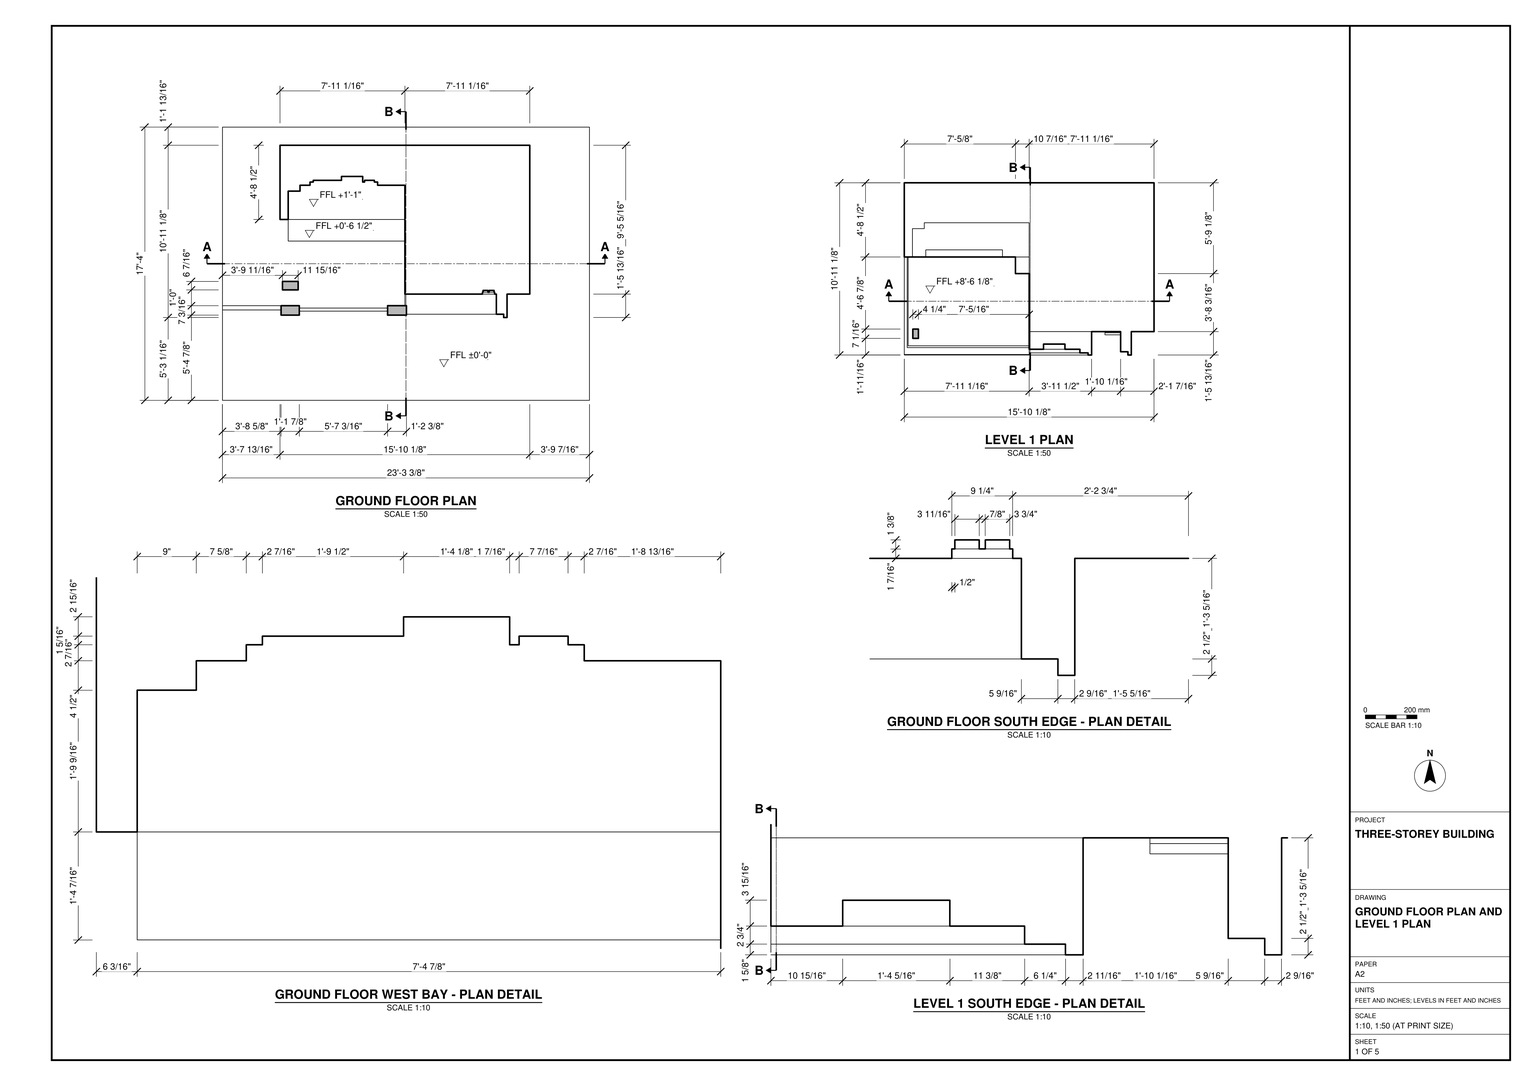
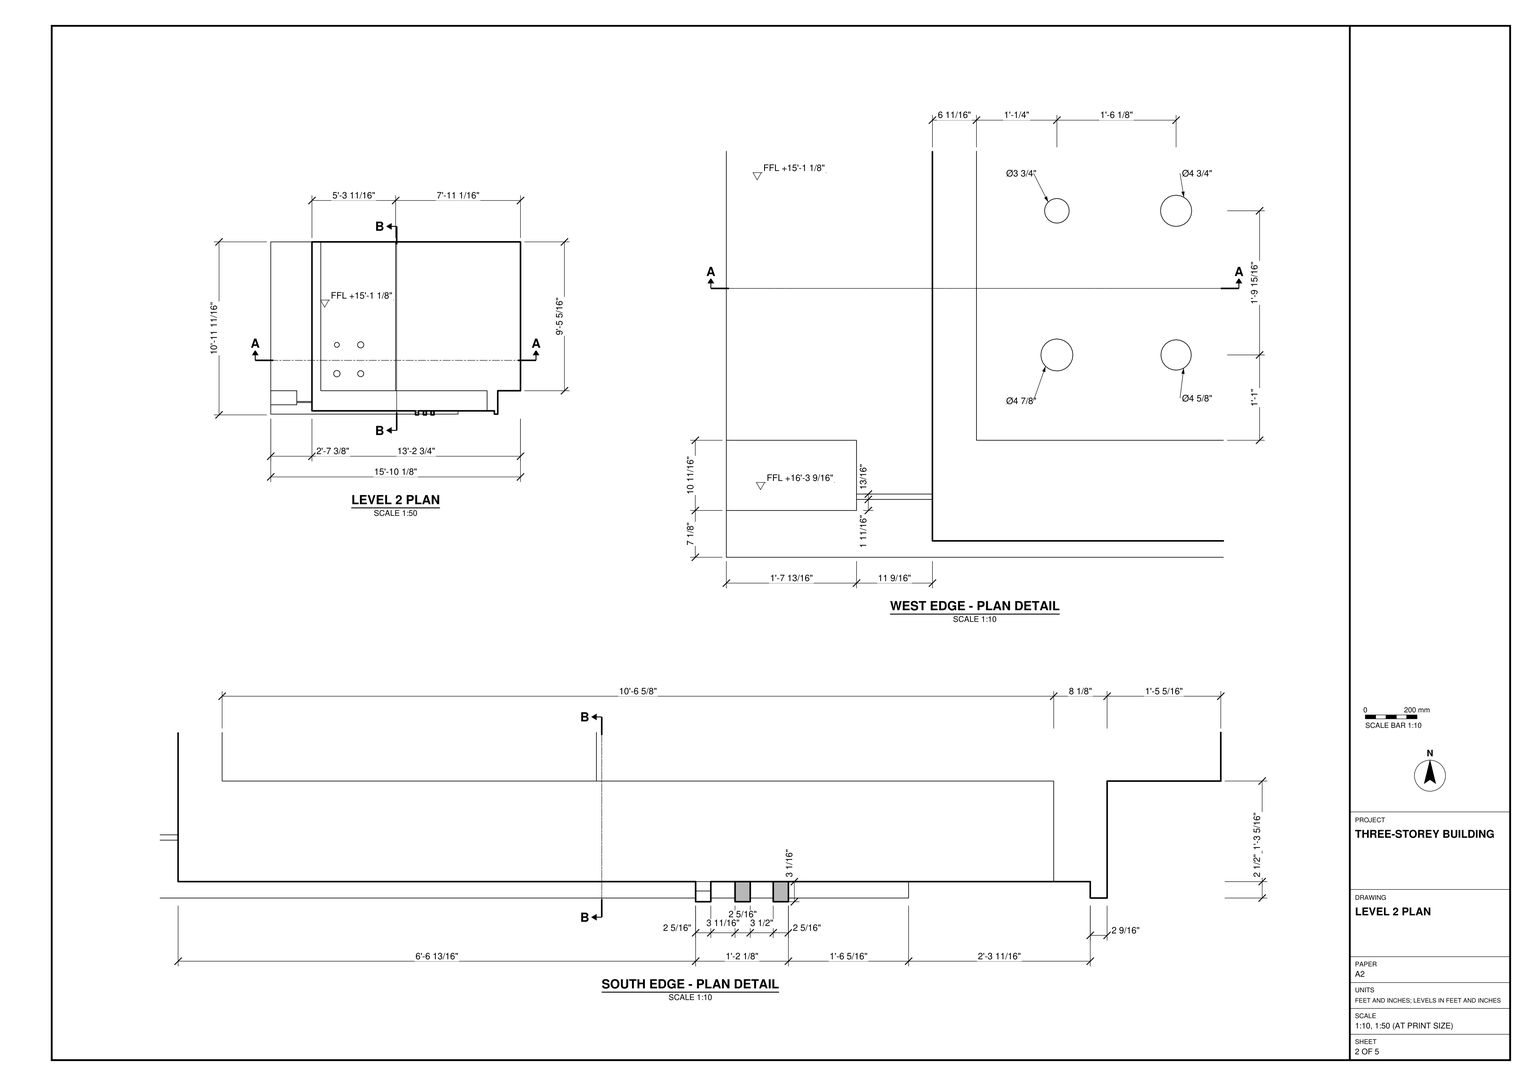
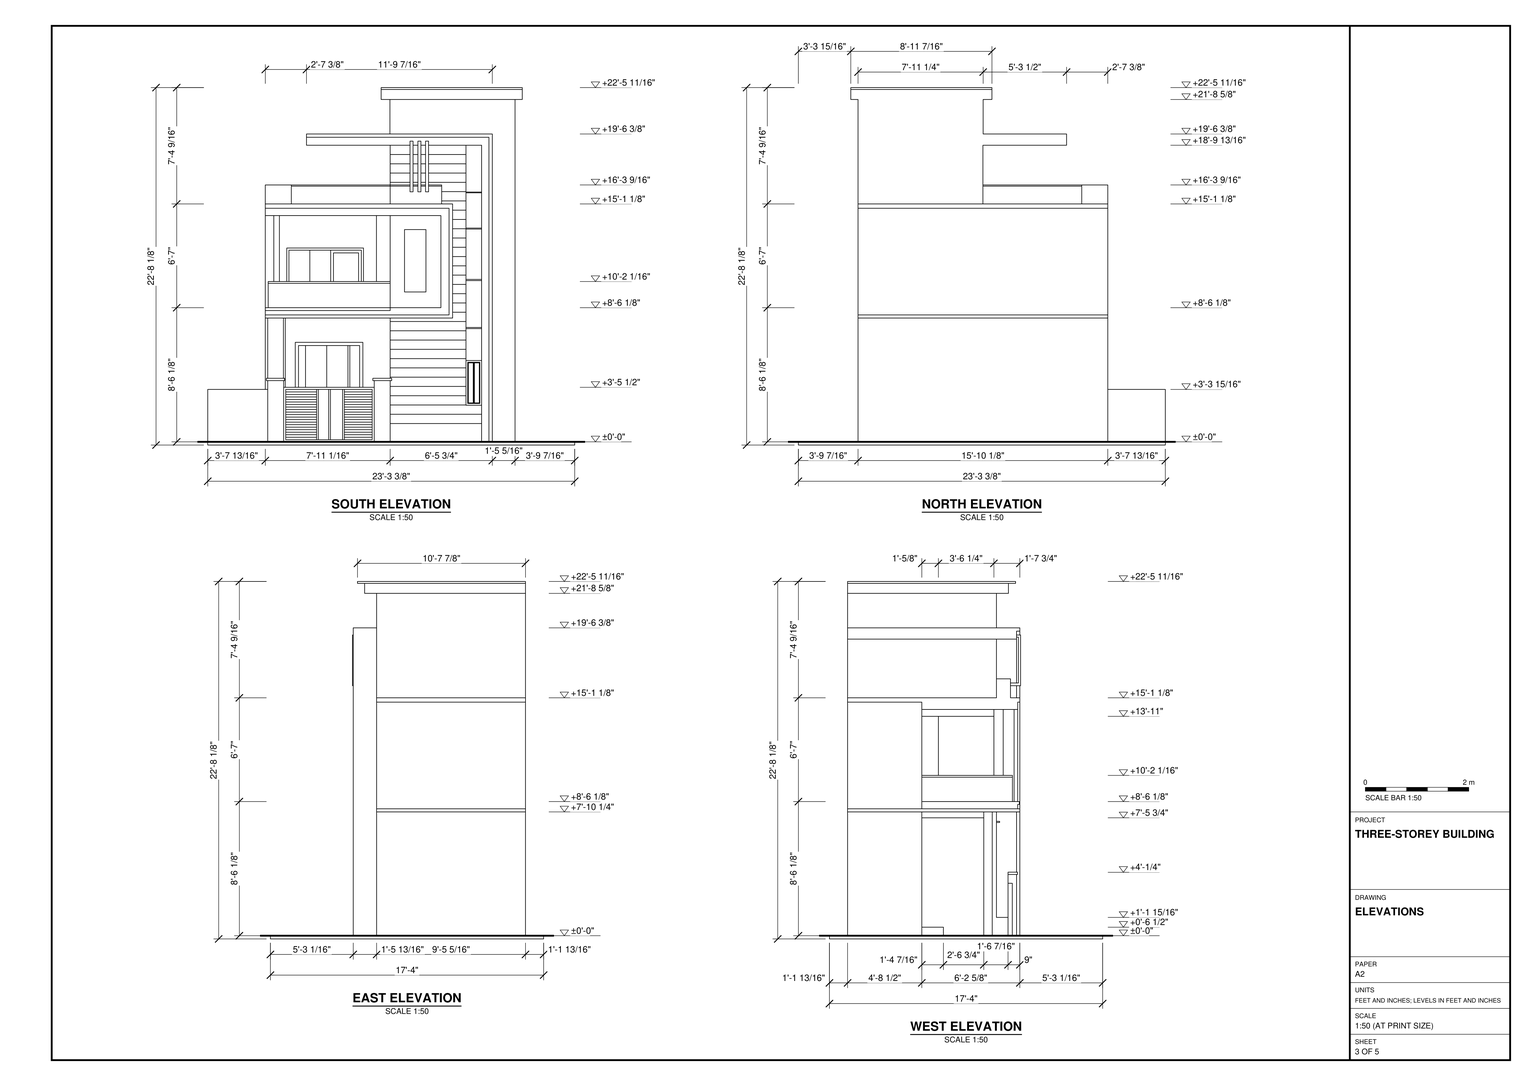
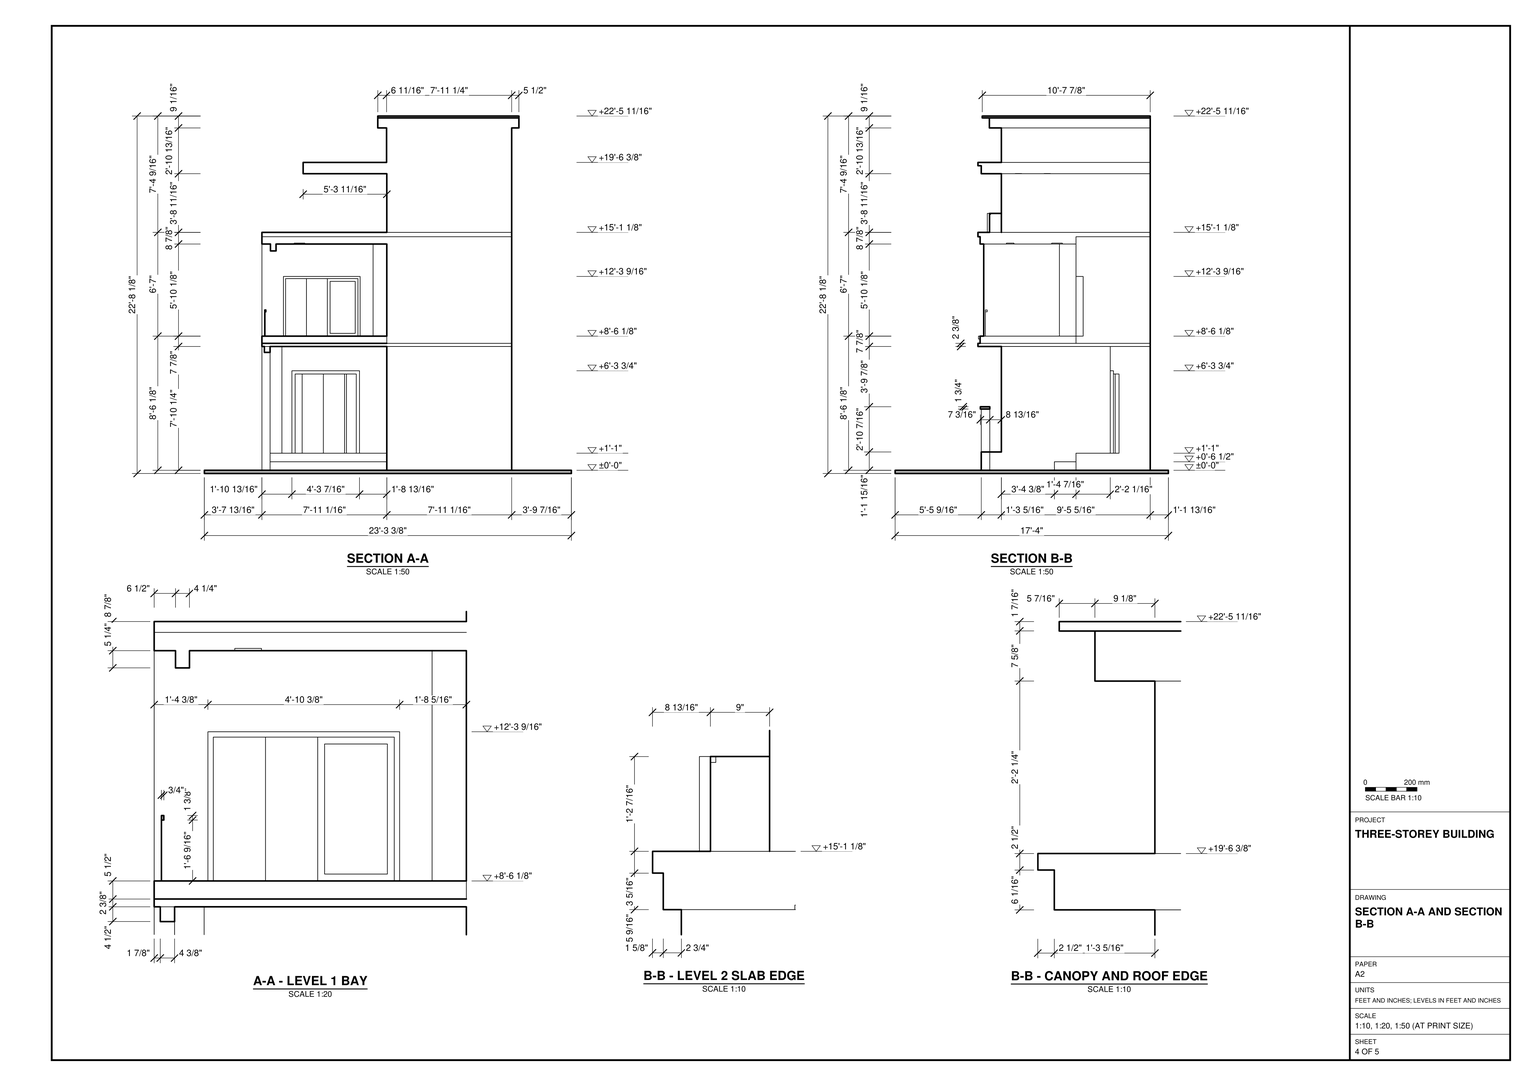
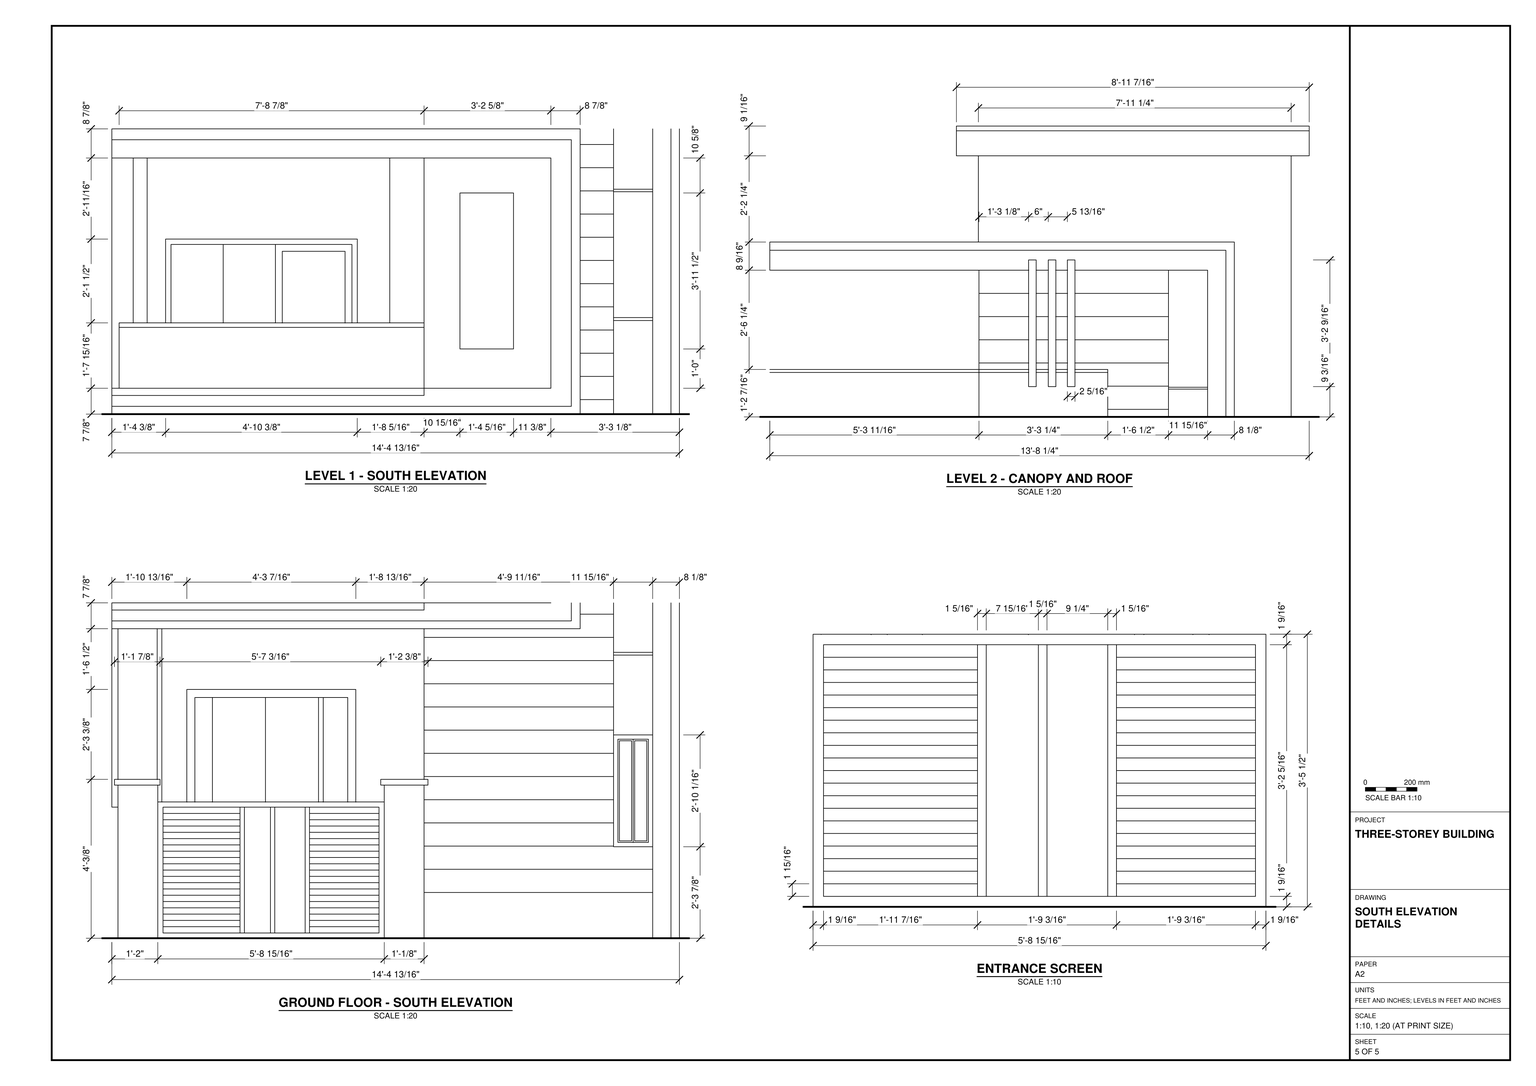
Build the three-storey building and its rectangular base in SketchUp using task_files/diagram_01.pdf. Work in feet and inches. The overall model measures 23'-3 3/8" east to west, 17'-4" north to south and 22'-8 1/8" high. Set the ground floor at ±0'-0", Level 1 at +8'-6 1/8" and Level 2 at +15'-1 1/8".

Use the plans to position the building on the base, leaving the open area in front of the south entrance. Follow the enlarged details for the stepped outline of the ground-floor west bay and the changes in the south edge at each level. Give the walls, floor slabs and roof their drawn thicknesses. Model the slatted entrance gate between its posts, with the ground-floor opening set back behind it. Above the gate, form the recessed balcony with its low front wall, divided opening and projecting rectangular surround.

Use the south elevation to place the horizontal bands on the east bay and the slim vertical fins beneath the upper projecting frame. Keep the upper enclosed volume to the east, leaving the terrace to the west, and finish it with the projecting flat roof cap. Organise walls, slabs, roof and any furniture or joinery pieces as separate groups or components; use components for repeated parts. Any decor or loose items shown may be represented by suitable library components. Save one SketchUp model as output_files/three_storey_building_with_its_framed_south_balcony.skp.

# SketchUp Ruby script. Lengths in inches.
U = 1.inch
M = Sketchup.active_model
def pt(a) = Geom::Point3d.new(a.map { |v| v * U })
def face(e, loops, mat)
  f = e.add_face(loops[0].map { |a| pt(a) })
  loops[1..].each { |l| e.add_face(l.map { |a| pt(a) }).erase! }
  f.material = f.back_material = mat if mat
  f
end
# faces: each face lists its corners as indices into pts; further lists are holes
def faces(e, pts, list, mat = nil) = list.each { |f| face(e, (f[0].is_a?(Array) ? f : [f]).map { |l| l.map { |i| pts[i] } }, mat) }
# xy, xz, yz: faces in a plane at the given z, y or x. An outline is a flat list of corners, or four numbers for a rectangle; further outlines are holes
def ring(l) = l.size == 4 ? [[l[0], l[1]], [l[2], l[1]], [l[2], l[3]], [l[0], l[3]]] : l.each_slice(2).to_a
def flat(e, list, mat, &to3) = list.each { |f| face(e, (f[0].is_a?(Array) ? f : [f]).map { |l| ring(l).map { |u, v| to3.(u, v) } }, mat) }
def xy(e, z, list, mat = nil) = flat(e, list, mat) { |x, y| [x, y, z] }
def xz(e, y, list, mat = nil) = flat(e, list, mat) { |x, z| [x, y, z] }
def yz(e, x, list, mat = nil) = flat(e, list, mat) { |y, z| [x, y, z] }
def lines(e, pts, list) = list.each { |a, b| e.add_line(pt(pts[a]), pt(pts[b])) }
# prism: a flat outline (further loops are holes) pulled along v
def prism(e, loops, v, mat = nil)
  f = face(e, loops, mat); d = Geom::Vector3d.new(v.map { |x| x * U })
  f.pushpull(f.normal.samedirection?(d) ? d.length : -d.length)
end
def box(e, o, s, mat = nil) = prism(e, [[o, [o[0] + s[0], o[1], o[2]], [o[0] + s[0], o[1] + s[1], o[2]], [o[0], o[1] + s[1], o[2]]]], [0, 0, s[2]], mat)
def at(x, y, z, deg = 0) = Geom::Transformation.translation(pt([x, y, z])) * Geom::Transformation.rotation(ORIGIN, Z_AXIS, deg.degrees)
def axes(o, x, y, z) = Geom::Transformation.new([*x, 0, *y, 0, *z, 0, *pt(o).to_a, 1])
def part(name) = M.definitions.add(name)
# library, detail: a bought-in or finely detailed component or shape, given as its bounding box
def library(name, o, s) = part(name).tap { |d| box(d.entities, o, s) }
def detail(e, o, s) = box(e.add_group.entities, o, s)
def put(e, d, t, mat = nil) = e.add_instance(d, t).tap { |i| i.material = mat if mat }
def group(e, t, mat = nil) = e.add_group.tap { |g| g.transformation = t; g.material = mat if mat }.entities
root = M.entities
M.materials.add("[Color M05]").color = [114, 114, 114]
M.materials.add("[Color M06]").color = [86, 86, 86]
M.materials.add("[Color M09]").color = [0, 0, 0]
M.materials.add("[Mosaic Hexagonal Tile]").color = [73, 84, 96]
M.materials.add("[Translucent Glass Gray]").color = [128, 128, 128]
M.materials["[Translucent Glass Gray]"].alpha = 0.5
M.materials.add("[Wood Bamboo]").color = [211, 125, 50]
xy(root,0,[[0,0,279.375,208]])
xy(root,2.4375,[[[0,0,279.375,0,279.375,208,0,208,0,72.0625,57.8,72.0625,57.8,70.25,126.75,70.25,126.75,72.0625,138.875,72.0625,138.875,121.25,50.03,121.25,50.03,137.6875,43.8125,137.6875,43.8125,194.1875,233.9375,194.1875,233.9375,80.875,216.63,80.875,216.63,63.0625,214.0625,63.0625,214.0625,65.5625,126.75,65.5625,126.75,67.91,57.8,67.91,57.8,65.5625,45.68,65.5625,45.68,68.8125,0,68.8125],[45.68,84.08,57.61,90.52]],[214.0625,63.0625,214.0625,65.5625,138.875,65.5625,138.875,121.25,50.03,121.25,50.03,137.6875,43.8125,137.6875,43.8125,194.1875,233.9375,194.1875,233.9375,80.875,216.63,80.875,216.63,63.0625],[45.68,65.5625,57.8,65.5625,57.8,72.0625,0,72.0625,0,68.8125,45.68,68.8125]])
xy(root,4.03,[[84.17,67.91,92.1,69.08],[92.1,67.91,93.42,70.25],[93.42,67.91,102.67,69.08],[84.17,69.08,92.1,70.25],[93.42,69.08,102.67,70.25]])
xy(root,8.92,[[50.03,121.25,138.875,137.6875]])
xy(root,15.41,[[50.03,137.6875,138.875,137.6875,138.875,163.75,118.09,163.75,118.09,166.1875,115.64,166.1875,115.64,167.5,108.18,167.5,108.18,166.1875,106.74,166.1875,106.74,170.4375,90.59,170.4375,90.59,167.5,69.09,167.5,69.09,166.1875,66.64,166.1875,66.64,163.75,59.03,163.75,59.03,159.27,50.03,159.27]])
xy(root,16.37,[[138.875,65.5625,208.5,80.875]],"[Color M05]")
xy(root,31.62,[[197.9,80.875,207.18,82.3125]])
xy(root,32.08,[[198.37,82.3125,202.08,83.6875],[203.01,82.3125,206.71,83.6875]])
xy(root,42.35,[[84.17,67.91,92.1,69.08],[92.1,67.91,93.42,70.25],[93.42,67.91,102.67,69.08],[0,68.8125,45.68,72.0625],[84.17,69.08,92.1,70.25],
  [93.42,69.08,102.67,70.25]])
xy(root,43.9375,[[57.8,67.91,126.75,70.25]])
xy(root,49.0625,[[44.61,64.875,57.8,65.5625],[57.8,64.875,58.49,72.0625],[125.6875,64.875,126.75,72.0625],[126.75,64.875,138.875,65.5625],[138.875,64.875,140.0625,72.0625],
  [44.61,65.5625,45.68,72.0625],[45.68,65.5625,57.8,72.0625],[126.75,65.5625,138.875,72.0625]])
xy(root,50.8125,[[44.61,64.875,58.49,72.0625],[125.6875,64.875,140.0625,72.0625]])
xy(root,62.57,[[198.37,82.3125,202.08,83.6875],[203.01,82.3125,206.71,83.6875]])
xy(root,63.03,[[197.9,80.875,207.18,82.3125]])
xy(root,75.74,[[69.09,166.1875,69.09,167.5,90.59,167.5,90.59,170.4375,106.74,170.4375,106.74,166.1875],[108.18,166.1875,115.64,167.5]])
xy(root,78.2,[[66.64,163.75,118.09,166.1875]])
xy(root,88.65,[[196.58,78.4375,208.5,80.875]])
xy(root,89.49,[[196.58,78.4375,208.5,80.875]])
xy(root,92.1875,[[45.68,90.52,50.03,137.6875]],"[Color M06]")
xy(root,96.6875,[[43.8125,63.0625,43.8125,137.6875,45.68,137.6875,45.68,84.08,57.61,84.08,57.61,90.52,50.03,90.52,50.03,159.27,59.03,159.27,59.03,163.75,138.875,163.75,138.875,63.0625],[138.875,63.0625,186.41,80.875],[45.68,84.08,57.61,90.52]])
xy(root,99.0625,[[43.8125,63.0625,183.72,64.6875],[43.8125,64.6875,138.875,137.6875]])
xy(root,102.375,[[43.8125,63.4375,138.875,64.6875]])
xy(root,104.5625,[[43.8125,63.4375,138.875,63.4375,138.875,68.71,46.03,68.71,46.03,137.6875,43.8125,137.6875],[138.875,64.6875,177.5,67.4375],[[46.03,68.71,138.875,68.71,138.875,125.06,128.4375,125.06,128.4375,137.6875,46.03,137.6875],[50.3125,75.74,54.5625,82.8125]],[60.18,137.6875,61.82,143.125],[61.82,137.6875,77.72,143.125],
  [77.72,137.6875,93.61,143.125],[93.61,137.6875,116.92,142.375],[116.92,137.6875,118.56,143.125]])
xy(root,106.66,[[95.71,142.375,114.82,143.125]])
xy(root,116.54,[[149.81,67.4375,166.12,71.375]])
xy(root,123.11,[[46.03,68.71,46.75,137.6875],[46.75,68.71,138.875,70.08]])
xy(root,124.48,[[46.03,68.71,138.875,68.71,138.875,70.08,46.75,70.08,46.75,137.6875,46.03,137.6875]],"[Color M06]")
xy(root,125.2,[[196.58,80,208.5,80.875]])
xy(root,126.09,[[196.58,80,208.5,80.875]])
xy(root,146.27,[[95.71,142.375,114.82,143.125]])
xy(root,148.36,[[93.61,142.375,116.92,143.125]])
xy(root,150,[[60.18,137.6875,118.56,143.125]])
xy(root,164.04,[[149.81,67.4375,166.12,71.375]])
xy(root,164.42,[[196.58,78.5,208.5,80.875]])
xy(root,165.17,[[196.58,78.5,208.5,80.875]])
xy(root,169.4375,[[50.3125,82.8125,54.5625,137.6875]],"[Color M06]")
xy(root,174.6875,[[[43.8125,64.6875,43.8125,137.6875,50.3125,137.6875,50.3125,75.74,54.5625,75.74,54.5625,137.6875,91.5,137.6875,91.5,75.0625,138.875,75.0625,138.875,64.6875],[72.42,119.17,73.47,119.3125,74.45,119.72,75.29,120.36,75.94,121.2,76.35,122.18,76.48,123.23,76.35,124.29,75.94,125.27,75.29,126.11,74.45,126.75,73.47,127.16,72.42,127.3,71.37,127.16,70.39,126.75,69.55,126.11,68.9,125.27,68.5,124.29,68.36,123.23,68.5,122.18,68.9,121.2,69.55,120.36,70.39,119.72,71.37,119.3125]],[138.875,64.6875,177.5,67.4375],[[91.5,75.0625,91.5,137.6875,128.4375,137.6875,128.4375,125.06,138.875,125.06,138.875,75.0625],[108.08,84.72,108.82,84.82,109.51,85.11,110.11,85.56,110.57,86.16,110.85,86.85,110.95,87.6,110.85,88.34,110.57,89.04,110.11,89.63,109.51,90.09,108.82,90.375,108.08,90.47,107.33,90.375,106.64,90.09,106.04,89.63,105.59,89.04,105.3,88.34,105.2,87.6,105.3,86.85,105.59,86.16,106.04,85.56,106.64,85.11,107.33,84.82]],[50.3125,75.74,54.5625,82.8125]])
xy(root,175.375,[[108.08,84.72,107.33,84.82,106.64,85.11,106.04,85.56,105.59,86.16,105.3,86.85,105.2,87.6,105.3,88.34,105.59,89.04,106.04,89.63,106.64,90.09,107.33,90.375,108.08,90.47,108.82,90.375,109.51,90.09,110.11,89.63,110.57,89.04,110.85,88.34,110.95,87.6,110.85,86.85,110.57,86.16,110.11,85.56,109.51,85.11,108.82,84.82],[72.42,119.17,71.37,119.3125,70.39,119.72,69.55,120.36,68.9,121.2,68.5,122.18,68.36,123.23,68.5,124.29,68.9,125.27,69.55,126.11,70.39,126.75,71.37,127.16,72.42,127.3,73.47,127.16,74.45,126.75,75.29,126.11,75.94,125.27,76.35,124.29,76.48,123.23,76.35,122.18,75.94,121.2,75.29,120.36,74.45,119.72,73.47,119.3125]],"[Wood Bamboo]")
xy(root,180.25,[[43.8125,63.0625,183.72,64.6875]])
xy(root,183.5625,[[43.8125,63.0625,186.41,63.0625,186.41,80.875,178.1,80.875,178.1,71.875,63.63,71.875,63.63,70.1875,43.8125,70.1875],[63.63,71.875,138.875,71.875,138.875,194.1875,43.8125,194.1875,43.8125,80.875,63.63,80.875]])
xy(root,192.03,[[196.58,79.625,208.5,80.875]])
xy(root,192.58,[[196.58,79.625,208.5,80.875]])
xy(root,192.78,[[153.98,62.5,156.3,71.875],[159.98,62.5,162.3,71.875],[165.8,62.5,168.11,71.875]])
xy(root,194.84,[[153.98,64.13,156.3,71.875],[159.98,64.13,162.3,71.875],[165.8,64.13,168.11,71.875]],"[Color M06]")
xy(root,197.1,[[63.63,71.875,138.875,72.6875]])
xy(root,198,[[43.8125,70.1875,63.63,80.875],[138.875,71.875,178.1,80.875]])
xy(root,198,[[63.63,71.875,138.875,72.6875]],"[Color M06]")
xy(root,228.23,[[75.1875,65.5625,75.1875,194.1875,81.89,194.1875,81.89,80.875,208.5,80.875,208.5,65.5625],[[81.89,80.875,138.875,194.1875],[94.14,91.43,94.77,91.51,95.36,91.76,95.86,92.14,96.25,92.65,96.49,93.24,96.57,93.87,96.49,94.5,96.25,95.09,95.86,95.59,95.36,95.98,94.77,96.22,94.14,96.31,93.51,96.22,92.92,95.98,92.41,95.59,92.03,95.09,91.78,94.5,91.7,93.87,91.78,93.24,92.03,92.65,92.41,92.14,92.92,91.76,93.51,91.51],[112.29,113.44,112.9,113.52,113.47,113.76,113.97,114.14,114.34,114.63,114.58,115.2,114.66,115.82,114.58,116.43,114.34,117.01,113.97,117.5,113.47,117.875,112.9,118.11,112.29,118.19,111.67,118.11,111.1,117.875,110.61,117.5,110.23,117.01,109.99,116.43,109.91,115.82,109.99,115.2,110.23,114.63,110.61,114.14,111.1,113.76,111.67,113.52],[112.29,91.56,112.88,91.63,113.44,91.87,113.92,92.23,114.29,92.71,114.52,93.27,114.6,93.87,114.52,94.47,114.29,95.02,113.92,95.5,113.44,95.87,112.88,96.1,112.29,96.18,111.6875,96.1,111.13,95.87,110.65,95.5,110.28,95.02,110.05,94.47,109.97,93.87,110.05,93.27,110.28,92.71,110.65,92.23,111.13,91.87,111.6875,91.63],[94.14,113.94,94.62,114.01,95.07,114.19,95.46,114.49,95.76,114.88,95.95,115.33,96.01,115.82,95.95,116.3,95.76,116.76,95.46,117.14,95.07,117.44,94.62,117.63,94.14,117.69,93.65,117.63,93.2,117.44,92.8125,117.14,92.51,116.76,92.33,116.3,92.26,115.82,92.33,115.33,92.51,114.88,92.8125,114.49,93.2,114.19,93.65,114.01]]])
xy(root,228.36,[[94.14,91.43,93.51,91.51,92.92,91.76,92.41,92.14,92.03,92.65,91.78,93.24,91.7,93.87,91.78,94.5,92.03,95.09,92.41,95.59,92.92,95.98,93.51,96.22,94.14,96.31,94.77,96.22,95.36,95.98,95.86,95.59,96.25,95.09,96.49,94.5,96.57,93.87,96.49,93.24,96.25,92.65,95.86,92.14,95.36,91.76,94.77,91.51],[112.29,91.56,111.6875,91.63,111.13,91.87,110.65,92.23,110.28,92.71,110.05,93.27,109.97,93.87,110.05,94.47,110.28,95.02,110.65,95.5,111.13,95.87,111.6875,96.1,112.29,96.18,112.88,96.1,113.44,95.87,113.92,95.5,114.29,95.02,114.52,94.47,114.6,93.87,114.52,93.27,114.29,92.71,113.92,92.23,113.44,91.87,112.88,91.63],[112.29,113.44,111.67,113.52,111.1,113.76,110.61,114.14,110.23,114.63,109.99,115.2,109.91,115.82,109.99,116.43,110.23,117.01,110.61,117.5,111.1,117.875,111.67,118.11,112.29,118.19,112.9,118.11,113.47,117.875,113.97,117.5,114.34,117.01,114.58,116.43,114.66,115.82,114.58,115.2,114.34,114.63,113.97,114.14,113.47,113.76,112.9,113.52],[94.14,113.94,93.65,114.01,93.2,114.19,92.8125,114.49,92.51,114.88,92.33,115.33,92.26,115.82,92.33,116.3,92.51,116.76,92.8125,117.14,93.2,117.44,93.65,117.63,94.14,117.69,94.62,117.63,95.07,117.44,95.46,117.14,95.76,116.76,95.95,116.3,96.01,115.82,95.95,115.33,95.76,114.88,95.46,114.49,95.07,114.19,94.62,114.01]],"[Wood Bamboo]")
xy(root,229.73,[[153.98,64.13,156.3,65.5625],[159.98,64.13,162.3,65.5625],[165.8,64.13,168.11,65.5625]])
xy(root,231.36,[[153.98,62.5,156.3,65.5625],[159.98,62.5,162.3,65.5625],[165.8,62.5,168.11,65.5625]],"[Color M06]")
xy(root,234.3,[[75.1875,63.0625,214.0625,65.5625]])
xy(root,236.8125,[[75.1875,63.0625,216.63,63.0625,216.63,80.875,138.69,80.875,138.69,194.1875,75.1875,194.1875]])
xy(root,263.07,[[132.01,71.75,132.01,194.1875,138.69,194.1875,138.69,80.875,233.9375,80.875,233.9375,194.1875,239.4375,194.1875,239.4375,71.75]])
xy(root,270.6875,[[132.01,66.3125,239.4375,71.75],[132.01,71.75,239.4375,194.1875]])
xy(root,272.125,[[132.01,66.3125,239.4375,71.75],[132.01,71.75,239.4375,194.1875]])
xz(root,0,[[0,0,279.375,2.4375]])
xz(root,62.5,[[153.98,192.78,156.3,231.36],[159.98,192.78,162.3,231.36],[165.8,192.78,168.11,231.36]],"[Color M06]")
xz(root,63.0625,[[214.0625,2.4375,216.63,2.4375,216.63,236.8125,75.1875,236.8125,75.1875,234.3,214.0625,234.3],[43.8125,96.6875,186.41,96.6875,186.41,183.5625,43.8125,183.5625,43.8125,180.25,183.72,180.25,183.72,99.0625,43.8125,99.0625]])
xz(root,63.4375,[[43.8125,102.375,138.875,104.5625]])
xz(root,64.13,[[153.98,194.84,156.3,229.73],[159.98,194.84,162.3,229.73],[165.8,194.84,168.11,229.73]])
xz(root,64.6875,[[43.8125,99.0625,183.72,99.0625,183.72,180.25,43.8125,180.25,43.8125,174.6875,177.5,174.6875,177.5,104.5625,138.875,104.5625,138.875,102.375,43.8125,102.375]])
xz(root,64.875,[[44.61,49.0625,58.49,50.8125],[125.6875,49.0625,140.0625,50.8125]])
xz(root,65.5625,[[45.68,2.4375,57.8,49.0625],[[208.5,2.4375,214.0625,2.4375,214.0625,234.3,75.1875,234.3,75.1875,228.23,208.5,228.23],[153.98,229.73,156.3,231.36]],[126.75,2.4375,138.875,49.0625]])
xz(root,65.5625,[[138.875,2.4375,208.5,16.37]],"[Color M05]")
xz(root,66.3125,[[132.01,270.6875,239.4375,272.125]])
xz(root,67.4375,[[[138.875,104.5625,177.5,174.6875],[149.81,116.54,166.12,164.04]]])
xz(root,67.91,[[[57.8,2.4375,126.75,43.9375],[59.39,4.03,125.16,42.35]],[82.84,4.03,84.17,42.35],[92.1,4.03,93.42,42.35],[102.67,4.03,104,42.35]],"[Color M09]")
xz(root,67.91,[[59.39,4.03,82.84,5.94],[104,4.03,125.16,5.94],[59.39,5.94,82.84,7.86],[104,5.94,125.16,7.86],[59.39,7.86,82.84,9.78],
  [104,7.86,125.16,9.78],[59.39,9.78,82.84,11.69],[104,9.78,125.16,11.69],[59.39,11.69,82.84,13.61],[104,11.69,125.16,13.61],
  [59.39,13.61,82.84,15.52],[104,13.61,125.16,15.52],[59.39,15.52,82.84,17.4375],[104,15.52,125.16,17.4375],[59.39,17.4375,82.84,19.36],
  [104,17.4375,125.16,19.36],[59.39,19.36,82.84,21.27],[104,19.36,125.16,21.27],[59.39,21.27,82.84,23.1875],[104,21.27,125.16,23.1875],
  [59.39,23.1875,82.84,25.1],[104,23.1875,125.16,25.1],[59.39,25.1,82.84,27.02],[104,25.1,125.16,27.02],[59.39,27.02,82.84,28.9375],
  [104,27.02,125.16,28.9375],[59.39,28.9375,82.84,30.85],[104,28.9375,125.16,30.85],[59.39,30.85,82.84,32.77],[104,30.85,125.16,32.77],
  [59.39,32.77,82.84,34.68],[104,32.77,125.16,34.68],[59.39,34.68,82.84,36.6],[104,34.68,125.16,36.6],[59.39,36.6,82.84,38.52],
  [104,36.6,125.16,38.52],[59.39,38.52,82.84,40.43],[104,38.52,125.16,40.43],[59.39,40.43,82.84,42.35],[104,40.43,125.16,42.35]],"[Wood Bamboo]")
xz(root,68.71,[[46.03,123.11,138.875,124.48]],"[Color M06]")
xz(root,68.71,[[46.03,104.5625,138.875,123.11]],"[Translucent Glass Gray]")
xz(root,68.8125,[[0,2.4375,45.68,42.35]])
xz(root,69.08,[[84.17,4.03,92.1,42.35],[93.42,4.03,102.67,42.35]],"[Translucent Glass Gray]")
xz(root,70.08,[[46.75,123.11,138.875,124.48]])
xz(root,70.1875,[[43.8125,183.5625,63.63,198]])
xz(root,70.25,[[[57.8,2.4375,126.75,43.9375],[84.17,4.03,102.67,42.35]],[92.1,4.03,93.42,42.35]])
xz(root,71.375,[[149.81,116.54,166.12,164.04]],"[Mosaic Hexagonal Tile]")
xz(root,71.75,[[132.01,263.07,239.4375,270.6875]])
xz(root,71.875,[[138.875,197.1,178.1,198]])
xz(root,71.875,[[[138.875,183.5625,178.1,197.1],[153.98,192.78,156.3,194.84]],[63.63,197.1,138.875,198]],"[Color M06]")
xz(root,71.875,[[63.63,183.5625,138.875,197.1]],"[Translucent Glass Gray]")
xz(root,72.0625,[[0,2.4375,0,42.35,45.68,42.35,45.68,49.0625,57.8,49.0625,57.8,2.4375],[126.75,2.4375,138.875,49.0625],[44.61,49.0625,58.49,50.8125],[125.6875,49.0625,140.0625,50.8125]])
xz(root,72.6875,[[63.63,197.1,138.875,198]])
xz(root,75.74,[[50.3125,104.5625,54.5625,174.6875]],"[Color M06]")
xz(root,78.4375,[[196.58,88.65,208.5,89.49]])
xz(root,78.5,[[196.58,164.42,208.5,165.17]])
xz(root,79.625,[[196.58,192.03,208.5,192.58]])
xz(root,80,[[196.58,125.2,208.5,126.09]])
xz(root,80.875,[[[196.58,30.29,208.5,64.36],[197.9,31.62,207.18,63.03]],[43.8125,183.5625,63.63,198],[138.875,183.5625,178.1,185.86],[138.875,185.86,178.1,192.92],[138.875,192.92,178.1,198]])
xz(root,80.875,[[196.58,64.36,208.5,88.65],[196.58,89.49,208.5,125.2],[196.58,126.09,208.5,164.42],[196.58,165.17,208.5,192.03],[196.58,192.58,208.5,228.23]],"[Translucent Glass Gray]")
xz(root,80.875,[[216.63,2.4375,233.9375,2.4375,233.9375,263.07,138.69,263.07,138.69,236.8125,216.63,236.8125],[138.875,16.37,208.5,23.43],[138.875,23.43,208.5,23.43,208.5,30.29,196.58,30.29,196.58,30.49,138.875,30.49],[138.875,30.49,196.58,37.55],[138.875,37.55,196.58,44.62],
  [138.875,44.62,196.58,51.68],[138.875,51.68,196.58,58.74],[138.875,58.74,196.58,65.8],[138.875,65.8,196.58,72.86],[138.875,72.86,196.58,79.93],
  [138.875,79.93,196.58,86.99],[138.875,86.99,196.58,94.05],[138.875,94.05,196.58,94.05,196.58,101.11,186.41,101.11,186.41,96.6875,138.875,96.6875],[186.41,101.11,196.58,108.17],[186.41,108.17,196.58,115.24],
  [186.41,115.24,196.58,122.3],[186.41,122.3,196.58,129.36],[186.41,129.36,196.58,136.42],[186.41,136.42,196.58,143.49],[186.41,143.49,196.58,150.55],
  [186.41,150.55,196.58,157.61],[186.41,157.61,196.58,164.67],[186.41,164.67,196.58,171.73],[186.41,171.73,196.58,178.8],[186.41,178.8,196.58,178.8,196.58,185.86,178.1,185.86,178.1,183.5625,186.41,183.5625],
  [178.1,185.86,196.58,192.92],[178.1,192.92,196.58,192.92,196.58,199.98,138.875,199.98,138.875,198,178.1,198],[138.875,199.98,196.58,207.05],[138.875,207.05,196.58,214.11],[138.875,214.11,196.58,221.17],
  [138.875,221.17,196.58,228.23]],"[Wood Bamboo]")
xz(root,82.3125,[[[197.9,31.62,202.54,63.03],[198.37,32.08,202.08,62.57]],[[202.54,31.62,207.18,63.03],[203.01,32.08,206.71,62.57]]])
xz(root,82.8125,[[50.3125,169.4375,54.5625,174.6875]])
xz(root,82.8125,[[50.3125,104.5625,54.5625,169.4375]],"[Color M06]")
xz(root,83.6875,[[198.37,32.08,202.08,62.57],[203.01,32.08,206.71,62.57]])
xz(root,84.08,[[45.68,2.4375,57.61,96.6875]],"[Color M06]")
xz(root,90.52,[[45.68,92.1875,50.03,96.6875]])
xz(root,90.52,[[45.68,2.4375,45.68,92.1875,50.03,92.1875,50.03,96.6875,57.61,96.6875,57.61,2.4375]],"[Color M06]")
xz(root,121.25,[[50.03,2.4375,138.875,8.92]])
xz(root,125.06,[[128.4375,104.5625,138.875,174.6875]])
xz(root,137.6875,[[43.8125,2.4375,50.03,2.4375,50.03,92.1875,45.68,92.1875,45.68,96.6875,43.8125,96.6875],[50.03,8.92,138.875,15.41],[45.68,92.1875,50.03,96.6875],[43.8125,99.0625,138.875,104.5625],[43.8125,104.5625,46.03,104.5625,46.03,124.48,46.75,124.48,46.75,123.11,46.03,123.11,46.03,104.5625,60.18,104.5625,60.18,150,118.56,150,118.56,104.5625,128.4375,104.5625,128.4375,174.6875,54.5625,174.6875,54.5625,169.4375,50.3125,169.4375,50.3125,174.6875,43.8125,174.6875]])
xz(root,142.375,[[[93.61,104.5625,116.92,148.36],[95.71,106.66,114.82,146.27]]])
xz(root,143.125,[[60.18,104.5625,61.82,104.5625,61.82,148.36,116.92,148.36,116.92,104.5625,118.56,104.5625,118.56,150,60.18,150],[61.82,104.5625,77.72,148.36]])
xz(root,143.125,[[95.71,106.66,114.82,146.27]],"[Translucent Glass Gray]")
xz(root,143.125,[[77.72,104.5625,93.61,148.36]],"[Wood Bamboo]")
xz(root,159.27,[[50.03,15.41,59.03,96.6875]])
xz(root,163.75,[[59.03,15.41,66.64,15.41,66.64,78.2,118.09,78.2,118.09,15.41,138.875,15.41,138.875,96.6875,59.03,96.6875]])
xz(root,166.1875,[[66.64,15.41,69.09,15.41,69.09,75.74,115.64,75.74,115.64,15.41,118.09,15.41,118.09,78.2,66.64,78.2],[106.74,15.41,108.18,75.74]])
xz(root,167.5,[[69.09,15.41,74.43,75.74],[108.18,15.41,115.64,75.74]],"[Translucent Glass Gray]")
xz(root,167.5,[[74.43,15.41,90.59,75.74]],"[Wood Bamboo]")
xz(root,170.4375,[[90.59,15.41,106.74,75.74]],"[Wood Bamboo]")
xz(root,194.1875,[[43.8125,2.4375,233.9375,96.6875],[43.8125,96.6875,233.9375,99.0625],[43.8125,99.0625,233.9375,180.25],[43.8125,180.25,233.9375,183.5625],[138.875,183.5625,138.875,228.23,75.1875,228.23,75.1875,236.8125,138.69,236.8125,138.69,263.07,132.01,263.07,132.01,270.6875,239.4375,270.6875,239.4375,263.07,233.9375,263.07,233.9375,183.5625],
  [132.01,270.6875,239.4375,272.125]])
xz(root,208,[[0,0,279.375,2.4375]])
yz(root,0,[[0,0,208,2.4375],[68.8125,2.4375,72.0625,42.35]])
yz(root,43.8125,[[137.6875,2.4375,194.1875,96.6875],[63.0625,96.6875,194.1875,99.0625],[64.6875,99.0625,64.6875,102.375,63.4375,102.375,63.4375,104.5625,137.6875,104.5625,137.6875,99.0625],[137.6875,99.0625,194.1875,180.25],[64.6875,174.6875,64.6875,180.25,63.0625,180.25,63.0625,183.5625,70.1875,183.5625,70.1875,198,80.875,198,80.875,183.5625,194.1875,183.5625,194.1875,180.25,137.6875,180.25,137.6875,174.6875]])
yz(root,44.61,[[64.875,49.0625,72.0625,50.8125]])
yz(root,45.68,[[65.5625,2.4375,65.5625,49.0625,72.0625,49.0625,72.0625,42.35,68.8125,42.35,68.8125,2.4375]])
yz(root,45.68,[[84.08,2.4375,90.52,96.6875],[90.52,92.1875,137.6875,96.6875]],"[Color M06]")
yz(root,46.03,[[68.71,123.11,137.6875,124.48]],"[Color M06]")
yz(root,46.03,[[68.71,104.5625,137.6875,123.11]],"[Translucent Glass Gray]")
yz(root,46.75,[[70.08,123.11,137.6875,124.48]],"[Color M06]")
yz(root,50.03,[[121.25,2.4375,137.6875,8.92],[137.6875,15.41,159.27,96.6875]])
yz(root,50.03,[[90.52,92.1875,137.6875,96.6875]],"[Color M06]")
yz(root,50.3125,[[75.74,104.5625,82.8125,174.6875],[82.8125,169.4375,137.6875,174.6875]],"[Color M06]")
yz(root,54.5625,[[75.74,104.5625,82.8125,174.6875],[82.8125,169.4375,137.6875,174.6875]],"[Color M06]")
yz(root,57.61,[[84.08,2.4375,90.52,96.6875]],"[Color M06]")
yz(root,57.8,[[65.5625,2.4375,67.91,2.4375,67.91,43.9375,70.25,43.9375,70.25,2.4375,72.0625,2.4375,72.0625,49.0625,65.5625,49.0625],[67.91,2.4375,70.25,43.9375]])
yz(root,58.49,[[64.875,49.0625,72.0625,50.8125]])
yz(root,59.03,[[159.27,15.41,163.75,96.6875]])
yz(root,60.18,[[137.6875,104.5625,143.125,150]])
yz(root,63.63,[[70.1875,183.5625,71.875,198],[71.875,183.5625,80.875,183.5625,80.875,198,72.6875,198,72.6875,197.1,71.875,197.1],[71.875,197.1,72.6875,198]])
yz(root,66.64,[[163.75,15.41,166.1875,78.2]])
yz(root,69.09,[[166.1875,15.41,167.5,75.74]])
yz(root,75.1875,[[65.5625,228.23,65.5625,234.3,63.0625,234.3,63.0625,236.8125,194.1875,236.8125,194.1875,228.23]])
yz(root,84.17,[[67.91,4.03,69.08,42.35],[69.08,4.03,70.25,42.35]])
yz(root,90.59,[[167.5,15.41,170.4375,75.74]])
yz(root,92.1,[[67.91,4.03,69.08,42.35],[69.08,4.03,70.25,42.35]])
yz(root,93.42,[[67.91,4.03,69.08,42.35],[69.08,4.03,70.25,42.35]])
yz(root,93.61,[[142.375,104.5625,143.125,148.36]])
yz(root,95.71,[[142.375,106.66,143.125,146.27]])
yz(root,102.67,[[67.91,4.03,69.08,42.35],[69.08,4.03,70.25,42.35]])
yz(root,106.74,[[166.1875,15.41,170.4375,75.74]])
yz(root,108.18,[[166.1875,15.41,167.5,75.74]])
yz(root,114.82,[[142.375,106.66,143.125,146.27]])
yz(root,115.64,[[166.1875,15.41,167.5,75.74]])
yz(root,116.92,[[142.375,104.5625,143.125,148.36]])
yz(root,118.09,[[163.75,15.41,166.1875,78.2]])
yz(root,118.56,[[137.6875,104.5625,143.125,150]])
yz(root,125.6875,[[64.875,49.0625,72.0625,50.8125]])
yz(root,126.75,[[65.5625,2.4375,65.5625,49.0625,72.0625,49.0625,72.0625,2.4375,70.25,2.4375,70.25,43.9375,67.91,43.9375,67.91,2.4375]])
yz(root,128.4375,[[125.06,104.5625,137.6875,174.6875]])
yz(root,132.01,[[71.75,263.07,194.1875,270.6875],[66.3125,270.6875,194.1875,272.125]])
yz(root,138.69,[[80.875,236.8125,194.1875,263.07]])
yz(root,138.875,[[65.5625,2.4375,72.0625,16.37],[72.0625,2.4375,72.0625,16.37,80.875,16.37,80.875,96.6875,163.75,96.6875,163.75,15.41,137.6875,15.41,137.6875,8.92,121.25,8.92,121.25,2.4375],[65.5625,16.37,72.0625,49.0625],[63.4375,102.375,64.6875,104.5625],[67.4375,104.5625,67.4375,174.6875,125.06,174.6875,125.06,104.5625,68.71,104.5625,68.71,123.11,70.08,123.11,70.08,124.48,68.71,124.48,68.71,104.5625],
  [71.875,183.5625,71.875,197.1,72.6875,197.1,72.6875,198,80.875,198,80.875,183.5625],[80.875,183.5625,194.1875,228.23],[71.875,197.1,72.6875,198]])
yz(root,140.0625,[[64.875,49.0625,72.0625,50.8125]])
yz(root,149.81,[[67.4375,116.54,71.375,164.04]])
yz(root,153.98,[[62.5,192.78,62.5,231.36,65.5625,231.36,65.5625,229.73,64.13,229.73,64.13,194.84,71.875,194.84,71.875,192.78]],"[Color M06]")
yz(root,156.3,[[62.5,192.78,71.875,192.78,71.875,194.84,64.13,194.84,64.13,229.73,65.5625,229.73,65.5625,231.36,62.5,231.36]])
yz(root,159.98,[[62.5,192.78,62.5,231.36,65.5625,231.36,65.5625,229.73,64.13,229.73,64.13,194.84,71.875,194.84,71.875,192.78]],"[Color M06]")
yz(root,162.3,[[62.5,192.78,71.875,192.78,71.875,194.84,64.13,194.84,64.13,229.73,65.5625,229.73,65.5625,231.36,62.5,231.36]])
yz(root,165.8,[[62.5,192.78,62.5,231.36,65.5625,231.36,65.5625,229.73,64.13,229.73,64.13,194.84,71.875,194.84,71.875,192.78]],"[Color M06]")
yz(root,166.12,[[67.4375,116.54,71.375,164.04]])
yz(root,168.11,[[62.5,192.78,71.875,192.78,71.875,194.84,64.13,194.84,64.13,229.73,65.5625,229.73,65.5625,231.36,62.5,231.36]])
yz(root,177.5,[[64.6875,104.5625,67.4375,174.6875]])
yz(root,178.1,[[71.875,183.5625,80.875,198]])
yz(root,183.72,[[63.0625,99.0625,64.6875,180.25]])
yz(root,186.41,[[63.0625,96.6875,80.875,183.5625]])
yz(root,196.58,[[78.4375,88.65,80.875,89.49],[80,125.2,80.875,126.09],[78.5,164.42,80.875,165.17],[79.625,192.03,80.875,192.58]])
yz(root,197.9,[[80.875,31.62,82.3125,63.03]])
yz(root,198.37,[[82.3125,32.08,83.6875,62.57]])
yz(root,202.08,[[82.3125,32.08,83.6875,62.57]])
yz(root,203.01,[[82.3125,32.08,83.6875,62.57]])
yz(root,206.71,[[82.3125,32.08,83.6875,62.57]])
yz(root,207.18,[[80.875,31.62,82.3125,63.03]])
yz(root,208.5,[[65.5625,16.37,65.5625,228.23,80.875,228.23,80.875,192.58,79.625,192.58,79.625,192.03,80.875,192.03,80.875,165.17,78.5,165.17,78.5,164.42,80.875,164.42,80.875,126.09,80,126.09,80,125.2,80.875,125.2,80.875,89.49,78.4375,89.49,78.4375,88.65,80.875,88.65,80.875,16.37]])
yz(root,214.0625,[[63.0625,2.4375,65.5625,234.3]])
yz(root,216.63,[[63.0625,2.4375,80.875,236.8125]])
yz(root,233.9375,[[80.875,2.4375,194.1875,96.6875],[80.875,96.6875,194.1875,99.0625],[80.875,99.0625,194.1875,180.25],[80.875,180.25,194.1875,183.5625],[80.875,183.5625,194.1875,263.07]])
yz(root,239.4375,[[71.75,263.07,194.1875,270.6875],[66.3125,270.6875,194.1875,272.125]])
yz(root,279.375,[[0,0,208,2.4375]])
# 13 loose lines left out
p = [[108.08,84.72,174.6875],[107.33,84.82,174.6875],[107.33,84.82,175.375],[108.08,84.72,175.375],[108.82,84.82,174.6875],[108.82,84.82,175.375],
  [106.64,85.11,174.6875],[106.64,85.11,175.375],[109.51,85.11,174.6875],[109.51,85.11,175.375],[106.04,85.56,174.6875],[106.04,85.56,175.375],
  [110.11,85.56,174.6875],[110.11,85.56,175.375],[105.59,86.16,174.6875],[105.59,86.16,175.375],[110.57,86.16,174.6875],[110.57,86.16,175.375],
  [105.3,86.85,174.6875],[105.3,86.85,175.375],[110.85,86.85,174.6875],[110.85,86.85,175.375],[105.2,87.6,174.6875],[105.2,87.6,175.375],
  [110.95,87.6,174.6875],[110.95,87.6,175.375],[105.3,88.34,174.6875],[105.3,88.34,175.375],[110.85,88.34,174.6875],[110.85,88.34,175.375],
  [105.59,89.04,174.6875],[105.59,89.04,175.375],[110.57,89.04,174.6875],[110.57,89.04,175.375],[106.04,89.63,174.6875],[106.04,89.63,175.375],
  [110.11,89.63,174.6875],[110.11,89.63,175.375],[106.64,90.09,174.6875],[106.64,90.09,175.375],[109.51,90.09,174.6875],[109.51,90.09,175.375],
  [107.33,90.375,174.6875],[107.33,90.375,175.375],[108.82,90.375,174.6875],[108.82,90.375,175.375],[108.08,90.47,174.6875],[108.08,90.47,175.375],
  [72.42,119.17,174.6875],[71.37,119.3125,174.6875],[71.37,119.3125,175.375],[72.42,119.17,175.375],[73.47,119.3125,174.6875],[73.47,119.3125,175.375],
  [70.39,119.72,174.6875],[70.39,119.72,175.375],[74.45,119.72,174.6875],[74.45,119.72,175.375],[69.55,120.36,174.6875],[69.55,120.36,175.375],
  [75.29,120.36,174.6875],[75.29,120.36,175.375],[68.9,121.2,174.6875],[68.9,121.2,175.375],[75.94,121.2,174.6875],[75.94,121.2,175.375],
  [68.5,122.18,174.6875],[68.5,122.18,175.375],[76.35,122.18,174.6875],[76.35,122.18,175.375],[68.36,123.23,174.6875],[68.36,123.23,175.375],
  [76.48,123.23,174.6875],[76.48,123.23,175.375],[68.5,124.29,174.6875],[68.5,124.29,175.375],[76.35,124.29,174.6875],[76.35,124.29,175.375],
  [68.9,125.27,174.6875],[68.9,125.27,175.375],[75.94,125.27,174.6875],[75.94,125.27,175.375],[69.55,126.11,174.6875],[69.55,126.11,175.375],
  [75.29,126.11,174.6875],[75.29,126.11,175.375],[70.39,126.75,174.6875],[70.39,126.75,175.375],[74.45,126.75,174.6875],[74.45,126.75,175.375],
  [71.37,127.16,174.6875],[71.37,127.16,175.375],[73.47,127.16,174.6875],[73.47,127.16,175.375],[72.42,127.3,174.6875],[72.42,127.3,175.375],
  [94.14,91.43,228.23],[93.51,91.51,228.23],[93.51,91.51,228.36],[94.14,91.43,228.36],[94.77,91.51,228.23],[94.77,91.51,228.36],
  [92.92,91.76,228.23],[92.92,91.76,228.36],[95.36,91.76,228.23],[95.36,91.76,228.36],[111.6875,91.63,228.23],[111.13,91.87,228.23],
  [111.13,91.87,228.36],[111.6875,91.63,228.36],[112.29,91.56,228.23],[112.29,91.56,228.36],[112.88,91.63,228.23],[112.88,91.63,228.36],
  [113.44,91.87,228.23],[113.44,91.87,228.36],[92.41,92.14,228.23],[92.41,92.14,228.36],[95.86,92.14,228.23],[95.86,92.14,228.36],
  [110.65,92.23,228.23],[110.65,92.23,228.36],[113.92,92.23,228.23],[113.92,92.23,228.36],[92.03,92.65,228.23],[92.03,92.65,228.36],
  [96.25,92.65,228.23],[96.25,92.65,228.36],[110.28,92.71,228.23],[110.28,92.71,228.36],[114.29,92.71,228.23],[114.29,92.71,228.36],
  [91.78,93.24,228.23],[91.78,93.24,228.36],[96.49,93.24,228.23],[96.49,93.24,228.36],[110.05,93.27,228.23],[110.05,93.27,228.36],
  [114.52,93.27,228.23],[114.52,93.27,228.36],[91.7,93.87,228.23],[91.7,93.87,228.36],[96.57,93.87,228.23],[96.57,93.87,228.36],
  [109.97,93.87,228.23],[109.97,93.87,228.36],[114.6,93.87,228.23],[114.6,93.87,228.36],[91.78,94.5,228.23],[91.78,94.5,228.36],
  [96.49,94.5,228.23],[96.49,94.5,228.36],[110.05,94.47,228.23],[110.05,94.47,228.36],[114.52,94.47,228.23],[114.52,94.47,228.36],
  [92.03,95.09,228.23],[92.03,95.09,228.36],[96.25,95.09,228.23],[96.25,95.09,228.36],[110.28,95.02,228.23],[110.28,95.02,228.36],
  [114.29,95.02,228.23],[114.29,95.02,228.36],[110.65,95.5,228.23],[110.65,95.5,228.36],[113.92,95.5,228.23],[113.92,95.5,228.36],
  [92.41,95.59,228.23],[92.41,95.59,228.36],[95.86,95.59,228.23],[95.86,95.59,228.36],[111.13,95.87,228.23],[111.13,95.87,228.36],
  [113.44,95.87,228.23],[113.44,95.87,228.36],[92.92,95.98,228.23],[92.92,95.98,228.36],[95.36,95.98,228.23],[95.36,95.98,228.36],
  [111.6875,96.1,228.23],[111.6875,96.1,228.36],[112.88,96.1,228.23],[112.88,96.1,228.36],[93.51,96.22,228.23],[93.51,96.22,228.36],
  [94.77,96.22,228.23],[94.77,96.22,228.36],[112.29,96.18,228.23],[112.29,96.18,228.36],[94.14,96.31,228.23],[94.14,96.31,228.36],
  [112.29,113.44,228.23],[111.67,113.52,228.23],[111.67,113.52,228.36],[112.29,113.44,228.36],[112.9,113.52,228.23],[112.9,113.52,228.36],
  [111.1,113.76,228.23],[111.1,113.76,228.36],[113.47,113.76,228.23],[113.47,113.76,228.36],[110.61,114.14,228.23],[110.61,114.14,228.36],
  [113.97,114.14,228.23],[113.97,114.14,228.36],[94.14,113.94,228.23],[93.65,114.01,228.23],[93.65,114.01,228.36],[94.14,113.94,228.36],
  [94.62,114.01,228.23],[94.62,114.01,228.36],[93.2,114.19,228.23],[93.2,114.19,228.36],[95.07,114.19,228.23],[95.07,114.19,228.36],
  [110.23,114.63,228.23],[110.23,114.63,228.36],[114.34,114.63,228.23],[114.34,114.63,228.36],[92.8125,114.49,228.23],[92.8125,114.49,228.36],
  [95.46,114.49,228.23],[95.46,114.49,228.36],[92.51,114.88,228.23],[92.51,114.88,228.36],[95.76,114.88,228.23],[95.76,114.88,228.36],
  [109.99,115.2,228.23],[109.99,115.2,228.36],[114.58,115.2,228.23],[114.58,115.2,228.36],[92.33,115.33,228.23],[92.33,115.33,228.36],
  [95.95,115.33,228.23],[95.95,115.33,228.36],[109.91,115.82,228.23],[109.91,115.82,228.36],[114.66,115.82,228.23],[114.66,115.82,228.36],
  [92.26,115.82,228.23],[92.26,115.82,228.36],[96.01,115.82,228.23],[96.01,115.82,228.36],[92.33,116.3,228.23],[92.33,116.3,228.36],
  [95.95,116.3,228.23],[95.95,116.3,228.36],[109.99,116.43,228.23],[109.99,116.43,228.36],[114.58,116.43,228.23],[114.58,116.43,228.36],
  [92.51,116.76,228.23],[92.51,116.76,228.36],[95.76,116.76,228.23],[95.76,116.76,228.36],[110.23,117.01,228.23],[110.23,117.01,228.36],
  [114.34,117.01,228.23],[114.34,117.01,228.36],[92.8125,117.14,228.23],[92.8125,117.14,228.36],[95.46,117.14,228.23],[95.46,117.14,228.36],
  [110.61,117.5,228.23],[110.61,117.5,228.36],[113.97,117.5,228.23],[113.97,117.5,228.36],[93.2,117.44,228.23],[93.2,117.44,228.36],
  [95.07,117.44,228.23],[95.07,117.44,228.36],[93.65,117.63,228.23],[93.65,117.63,228.36],[94.62,117.63,228.23],[94.62,117.63,228.36],
  [111.1,117.875,228.23],[111.1,117.875,228.36],[113.47,117.875,228.23],[113.47,117.875,228.36],[94.14,117.69,228.23],[94.14,117.69,228.36],
  [111.67,118.11,228.23],[111.67,118.11,228.36],[112.9,118.11,228.23],[112.9,118.11,228.36],[112.29,118.19,228.23],[112.29,118.19,228.36]]
faces(root,p,[[0,1,2,3],[4,0,3,5],[1,6,7,2],[8,4,5,9],[6,10,11,7],[12,8,9,13],[10,14,15,11],[16,12,13,17],
  [14,18,19,15],[20,16,17,21],[18,22,23,19],[24,20,21,25],[22,26,27,23],[28,24,25,29],[26,30,31,27],[32,28,29,33],
  [30,34,35,31],[36,32,33,37],[34,38,39,35],[40,36,37,41],[38,42,43,39],[44,40,41,45],[42,46,47,43],[46,44,45,47],
  [48,49,50,51],[52,48,51,53],[49,54,55,50],[56,52,53,57],[54,58,59,55],[60,56,57,61],[58,62,63,59],[64,60,61,65],
  [62,66,67,63],[68,64,65,69],[66,70,71,67],[72,68,69,73],[70,74,75,71],[76,72,73,77],[74,78,79,75],[80,76,77,81],
  [78,82,83,79],[84,80,81,85],[82,86,87,83],[88,84,85,89],[86,90,91,87],[92,88,89,93],[90,94,95,91],[94,92,93,95],
  [96,97,98,99],[100,96,99,101],[97,102,103,98],[104,100,101,105],[106,107,108,109],[110,106,109,111],[112,110,111,113],[114,112,113,115],
  [102,116,117,103],[118,104,105,119],[107,120,121,108],[122,114,115,123],[116,124,125,117],[126,118,119,127],[120,128,129,121],[130,122,123,131],
  [124,132,133,125],[134,126,127,135],[128,136,137,129],[138,130,131,139],[132,140,141,133],[142,134,135,143],[136,144,145,137],[146,138,139,147],
  [140,148,149,141],[150,142,143,151],[144,152,153,145],[154,146,147,155],[148,156,157,149],[158,150,151,159],[152,160,161,153],[162,154,155,163],
  [160,164,165,161],[166,162,163,167],[156,168,169,157],[170,158,159,171],[164,172,173,165],[174,166,167,175],[168,176,177,169],[178,170,171,179],
  [172,180,181,173],[182,174,175,183],[176,184,185,177],[186,178,179,187],[180,188,189,181],[188,182,183,189],[184,190,191,185],[190,186,187,191],
  [192,193,194,195],[196,192,195,197],[193,198,199,194],[200,196,197,201],[198,202,203,199],[204,200,201,205],[206,207,208,209],[210,206,209,211],
  [207,212,213,208],[214,210,211,215],[202,216,217,203],[218,204,205,219],[212,220,221,213],[222,214,215,223],[220,224,225,221],[226,222,223,227],
  [216,228,229,217],[230,218,219,231],[224,232,233,225],[234,226,227,235],[228,236,237,229],[238,230,231,239],[232,240,241,233],[242,234,235,243],
  [240,244,245,241],[246,242,243,247],[236,248,249,237],[250,238,239,251],[244,252,253,245],[254,246,247,255],[248,256,257,249],[258,250,251,259],
  [252,260,261,253],[262,254,255,263],[256,264,265,257],[266,258,259,267],[260,268,269,261],[270,262,263,271],[268,272,273,269],[274,270,271,275],
  [264,276,277,265],[278,266,267,279],[272,280,281,273],[280,274,275,281],[276,282,283,277],[284,278,279,285],[282,286,287,283],[286,284,285,287]])
